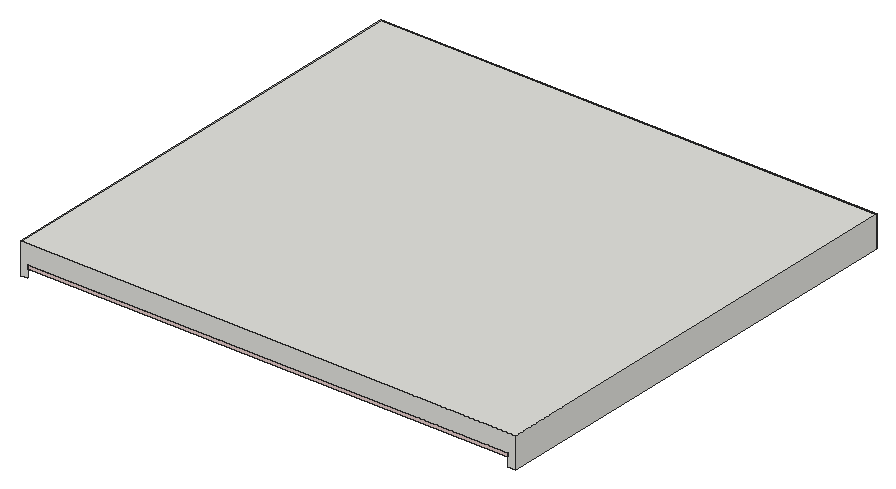
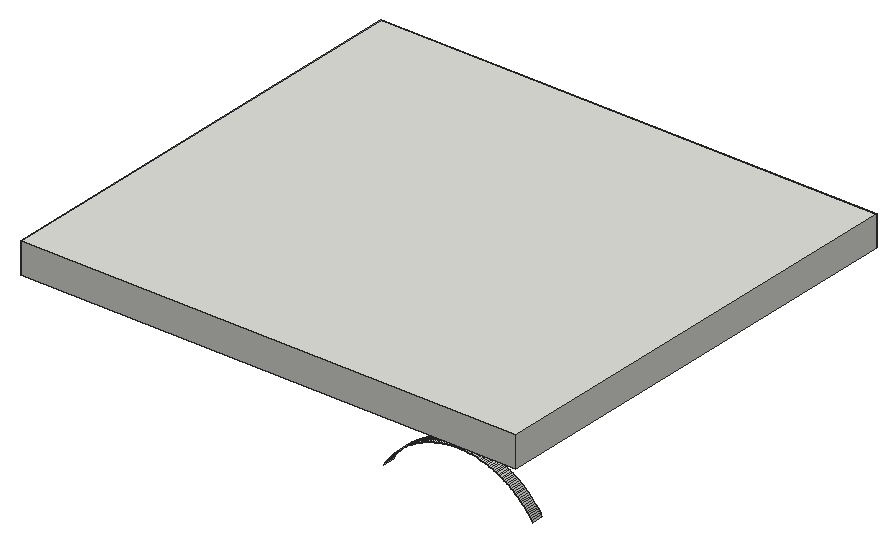
# SketchUp Ruby script. Lengths in inches.
U = 1.inch
M = Sketchup.active_model
def pt(a) = Geom::Point3d.new(a.map { |v| v * U })
def face(e, loops, mat)
  f = e.add_face(loops[0].map { |a| pt(a) })
  loops[1..].each { |l| e.add_face(l.map { |a| pt(a) }).erase! }
  f.material = f.back_material = mat if mat
  f
end
# faces: each face lists its corners as indices into pts; further lists are holes
def faces(e, pts, list, mat = nil) = list.each { |f| face(e, (f[0].is_a?(Array) ? f : [f]).map { |l| l.map { |i| pts[i] } }, mat) }
# xy, xz, yz: faces in a plane at the given z, y or x. An outline is a flat list of corners, or four numbers for a rectangle; further outlines are holes
def ring(l) = l.size == 4 ? [[l[0], l[1]], [l[2], l[1]], [l[2], l[3]], [l[0], l[3]]] : l.each_slice(2).to_a
def flat(e, list, mat, &to3) = list.each { |f| face(e, (f[0].is_a?(Array) ? f : [f]).map { |l| ring(l).map { |u, v| to3.(u, v) } }, mat) }
def xy(e, z, list, mat = nil) = flat(e, list, mat) { |x, y| [x, y, z] }
def xz(e, y, list, mat = nil) = flat(e, list, mat) { |x, z| [x, y, z] }
def yz(e, x, list, mat = nil) = flat(e, list, mat) { |y, z| [x, y, z] }
def lines(e, pts, list) = list.each { |a, b| e.add_line(pt(pts[a]), pt(pts[b])) }
# prism: a flat outline (further loops are holes) pulled along v
def prism(e, loops, v, mat = nil)
  f = face(e, loops, mat); d = Geom::Vector3d.new(v.map { |x| x * U })
  f.pushpull(f.normal.samedirection?(d) ? d.length : -d.length)
end
def box(e, o, s, mat = nil) = prism(e, [[o, [o[0] + s[0], o[1], o[2]], [o[0] + s[0], o[1] + s[1], o[2]], [o[0], o[1] + s[1], o[2]]]], [0, 0, s[2]], mat)
def at(x, y, z, deg = 0) = Geom::Transformation.translation(pt([x, y, z])) * Geom::Transformation.rotation(ORIGIN, Z_AXIS, deg.degrees)
def axes(o, x, y, z) = Geom::Transformation.new([*x, 0, *y, 0, *z, 0, *pt(o).to_a, 1])
def part(name) = M.definitions.add(name)
# library, detail: a bought-in or finely detailed component or shape, given as its bounding box
def library(name, o, s) = part(name).tap { |d| box(d.entities, o, s) }
def detail(e, o, s) = box(e.add_group.entities, o, s)
def put(e, d, t, mat = nil) = e.add_instance(d, t).tap { |i| i.material = mat if mat }
def group(e, t, mat = nil) = e.add_group.tap { |g| g.transformation = t; g.material = mat if mat }.entities
root = M.entities
M.materials.add("[0007_MistyRose]").color = [232, 207, 204]
M.materials.add("[0134_DimGray]").color = [105, 105, 105]
xy(root,122.125,[[77.27,180.253,114.094,204.253],[114.394,180.253,114.394,180.378,114.094,180.378,114.094,204.253,150.918,204.253,150.918,180.253],[150.918,180.253,150.918,204.253,187.741,204.253,187.741,183.815,169.329,183.815,169.329,180.253],[169.329,180.253,187.741,183.815],[188.041,180.253,208.642,180.378],
  [208.642,180.253,224.565,180.378],[187.741,180.378,224.565,204.253],[3.622,184.565,40.446,189.878],[40.446,184.565,77.27,204.253],[3.622,189.878,40.446,204.253]])
xy(root,127.75,[[3.435,0,3.435,93.375,3.622,204.253,3.622,189.878,40.446,189.878,40.446,184.565,77.27,184.565,77.27,180.253,114.094,180.253,114.094,180.378,114.394,180.378,114.394,180.253,169.329,180.253,169.329,183.815,187.741,183.815,187.741,180.378,224.565,180.378,224.565,0]])
xy(root,136.1875,[[0,0,228,207.6875]])
xz(root,0,[[0,122.125,3.435,122.125,3.435,127.75,224.565,127.75,224.565,122.125,228,122.125,228,136.1875,0,136.1875]])
xz(root,180.253,[[77.27,122.125,95.682,127.75],[95.682,122.125,114.094,127.75],[114.394,122.125,133.557,127.75],[133.557,122.125,150.918,127.75],[150.918,122.125,151.218,127.75],
  [151.218,122.125,169.329,127.75]])
xz(root,180.378,[[114.094,122.125,114.394,127.75],[187.741,122.125,188.041,127.75]])
xz(root,180.378,[[188.041,122.125,224.565,127.75]],"[0134_DimGray]")
xz(root,183.815,[[169.329,122.125,187.741,127.75]],"[0134_DimGray]")
xz(root,184.565,[[40.446,122.125,77.27,127.75]],"[0134_DimGray]")
xz(root,189.878,[[3.622,122.125,40.446,127.75]],"[0134_DimGray]")
xz(root,207.6875,[[0,122.125,228,136.1875]])
yz(root,0,[[0,122.125,207.6875,136.1875]])
yz(root,3.622,[[189.878,122.125,204.253,127.75]])
yz(root,40.446,[[184.565,122.125,189.878,127.75]])
yz(root,77.27,[[180.253,122.125,184.565,127.75]])
yz(root,114.094,[[180.253,122.125,180.378,127.75]])
yz(root,114.394,[[180.253,122.125,180.378,127.75]])
yz(root,169.329,[[180.253,122.125,183.815,127.75]])
yz(root,187.741,[[180.378,122.125,183.815,127.75]])
yz(root,228,[[0,122.125,207.6875,136.1875]])
p = [[6.197,184.565,90.119],[6.197,190.128,90.119],[6.615,190.128,90.765],[6.615,184.565,90.765],[74.277,184.565,90.765],[74.277,190.128,90.765],
  [74.695,190.128,90.119],[74.695,184.565,90.119],[7.046,190.128,91.403],[7.046,184.565,91.403],[73.847,184.565,91.403],[73.847,190.128,91.403],
  [7.488,190.128,92.033],[7.488,184.565,92.033],[73.404,184.565,92.033],[73.404,190.128,92.033],[7.942,190.128,92.654],[7.942,184.565,92.654],
  [72.95,184.565,92.654],[72.95,190.128,92.654],[8.408,190.128,93.266],[8.408,184.565,93.266],[72.484,184.565,93.266],[72.484,190.128,93.266],
  [8.886,190.128,93.869],[8.886,184.565,93.869],[72.006,184.565,93.869],[72.006,190.128,93.869],[9.375,190.128,94.464],[9.375,184.565,94.464],
  [71.517,184.565,94.464],[71.517,190.128,94.464],[9.875,190.128,95.048],[9.875,184.565,95.048],[71.017,184.565,95.048],[71.017,190.128,95.048],
  [10.386,190.128,95.624],[10.386,184.565,95.624],[70.506,184.565,95.624],[70.506,190.128,95.624],[10.908,190.128,96.189],[10.908,184.565,96.189],
  [69.984,184.565,96.189],[69.984,190.128,96.189],[11.441,190.128,96.744],[11.441,184.565,96.744],[69.452,184.565,96.744],[69.452,190.128,96.744],
  [11.984,190.128,97.29],[11.984,184.565,97.29],[68.909,184.565,97.29],[68.909,190.128,97.29],[12.537,190.128,97.824],[12.537,184.565,97.824],
  [68.355,184.565,97.824],[68.355,190.128,97.824],[13.1,190.128,98.349],[13.1,184.565,98.349],[67.792,184.565,98.349],[67.792,190.128,98.349],
  [13.673,190.128,98.862],[13.673,184.565,98.862],[67.219,184.565,98.862],[67.219,190.128,98.862],[14.256,190.128,99.365],[14.256,184.565,99.365],
  [66.636,184.565,99.365],[66.636,190.128,99.365],[14.848,190.128,99.856],[14.848,184.565,99.856],[66.044,184.565,99.856],[66.044,190.128,99.856],
  [15.45,190.128,100.336],[15.45,184.565,100.336],[65.442,184.565,100.336],[65.442,190.128,100.336],[16.06,190.128,100.804],[16.06,184.565,100.804],
  [64.832,184.565,100.804],[64.832,190.128,100.804],[16.679,190.128,101.261],[16.679,184.565,101.261],[64.213,184.565,101.261],[64.213,190.128,101.261],
  [17.307,190.128,101.706],[17.307,184.565,101.706],[63.585,184.565,101.706],[63.585,190.128,101.706],[17.943,190.128,102.139],[17.943,184.565,102.139],
  [62.949,184.565,102.139],[62.949,190.128,102.139],[18.588,190.128,102.56],[18.588,184.565,102.56],[62.305,184.565,102.56],[62.305,190.128,102.56],
  [19.24,190.128,102.969],[19.24,184.565,102.969],[61.653,184.565,102.969],[61.653,190.128,102.969],[19.899,190.128,103.365],[19.899,184.565,103.365],
  [60.993,184.565,103.365],[60.993,190.128,103.365],[20.566,190.128,103.748],[20.566,184.565,103.748],[60.326,184.565,103.748],[60.326,190.128,103.748],
  [21.241,190.128,104.119],[21.241,184.565,104.119],[59.652,184.565,104.119],[59.652,190.128,104.119],[21.922,190.128,104.477],[21.922,184.565,104.477],
  [58.97,184.565,104.477],[58.97,190.128,104.477],[22.61,190.128,104.822],[22.61,184.565,104.822],[58.283,184.565,104.822],[58.283,190.128,104.822],
  [23.304,190.128,105.154],[23.304,184.565,105.154],[57.588,184.565,105.154],[57.588,190.128,105.154],[24.004,190.128,105.473],[24.004,184.565,105.473],
  [56.888,184.565,105.473],[56.888,190.128,105.473],[24.711,190.128,105.778],[24.711,184.565,105.778],[56.181,184.565,105.778],[56.181,190.128,105.778],
  [25.423,190.128,106.07],[25.423,184.565,106.07],[55.469,184.565,106.07],[55.469,190.128,106.07],[26.14,190.128,106.348],[26.14,184.565,106.348],
  [54.752,184.565,106.348],[54.752,190.128,106.348],[26.863,190.128,106.612],[26.863,184.565,106.612],[54.029,184.565,106.612],[54.029,190.128,106.612],
  [27.59,190.128,106.863],[27.59,184.565,106.863],[53.302,184.565,106.863],[53.302,190.128,106.863],[28.322,190.128,107.1],[28.322,184.565,107.1],
  [52.57,184.565,107.1],[52.57,190.128,107.1],[29.059,190.128,107.323],[29.059,184.565,107.323],[51.833,184.565,107.323],[51.833,190.128,107.323],
  [29.799,190.128,107.532],[29.799,184.565,107.532],[51.093,184.565,107.532],[51.093,190.128,107.532],[30.544,190.128,107.727],[30.544,184.565,107.727],
  [50.349,184.565,107.727],[50.349,190.128,107.727],[31.292,190.128,107.908],[31.292,184.565,107.908],[49.601,184.565,107.908],[49.601,190.128,107.908],
  [32.043,190.128,108.075],[32.043,184.565,108.075],[48.849,184.565,108.075],[48.849,190.128,108.075],[32.797,190.128,108.227],[32.797,184.565,108.227],
  [48.095,184.565,108.227],[48.095,190.128,108.227],[33.554,190.128,108.365],[33.554,184.565,108.365],[47.338,184.565,108.365],[47.338,190.128,108.365],
  [34.314,190.128,108.489],[34.314,184.565,108.489],[46.579,184.565,108.489],[46.579,190.128,108.489],[35.075,190.128,108.598],[35.075,184.565,108.598],
  [45.817,184.565,108.598],[45.817,190.128,108.598],[35.839,190.128,108.692],[35.839,184.565,108.692],[45.053,184.565,108.692],[45.053,190.128,108.692],
  [36.604,190.128,108.773],[36.604,184.565,108.773],[44.288,184.565,108.773],[44.288,190.128,108.773],[37.371,190.128,108.838],[37.371,184.565,108.838],
  [38.139,190.128,108.889],[38.139,184.565,108.889],[42.753,184.565,108.889],[42.753,190.128,108.889],[43.521,190.128,108.838],[43.521,184.565,108.838],
  [38.907,190.128,108.926],[38.907,184.565,108.926],[39.677,190.128,108.948],[39.677,184.565,108.948],[40.446,190.128,108.955],[40.446,184.565,108.955],
  [40.746,190.128,108.952],[41.216,190.128,108.948],[41.216,184.565,108.948],[41.985,190.128,108.926],[41.985,184.565,108.926],[40.746,190.128,108.955]]
faces(root,p,[[0,1,2,3],[4,5,6,7],[3,2,8,9],[10,11,5,4],[9,8,12,13],[14,15,11,10],[13,12,16,17],[18,19,15,14],
  [17,16,20,21],[22,23,19,18],[21,20,24,25],[26,27,23,22],[25,24,28,29],[30,31,27,26],[29,28,32,33],[34,35,31,30],
  [33,32,36,37],[38,39,35,34],[37,36,40,41],[42,43,39,38],[41,40,44,45],[46,47,43,42],[45,44,48,49],[50,51,47,46],
  [49,48,52,53],[54,55,51,50],[53,52,56,57],[58,59,55,54],[57,56,60,61],[62,63,59,58],[61,60,64,65],[66,67,63,62],
  [65,64,68,69],[70,71,67,66],[69,68,72,73],[74,75,71,70],[73,72,76,77],[78,79,75,74],[77,76,80,81],[82,83,79,78],
  [81,80,84,85],[86,87,83,82],[85,84,88,89],[90,91,87,86],[89,88,92,93],[94,95,91,90],[93,92,96,97],[98,99,95,94],
  [97,96,100,101],[102,103,99,98],[101,100,104,105],[106,107,103,102],[105,104,108,109],[110,111,107,106],[109,108,112,113],[114,115,111,110],
  [113,112,116,117],[118,119,115,114],[117,116,120,121],[122,123,119,118],[121,120,124,125],[126,127,123,122],[125,124,128,129],[130,131,127,126],
  [129,128,132,133],[134,135,131,130],[133,132,136,137],[138,139,135,134],[137,136,140,141],[142,143,139,138],[141,140,144,145],[146,147,143,142],
  [145,144,148,149],[150,151,147,146],[149,148,152,153],[154,155,151,150],[153,152,156,157],[158,159,155,154],[157,156,160,161],[162,163,159,158],
  [161,160,164,165],[166,167,163,162],[165,164,168,169],[170,171,167,166],[169,168,172,173],[174,175,171,170],[173,172,176,177],[178,179,175,174],
  [177,176,180,181],[182,183,179,178],[181,180,184,185],[186,187,183,182],[185,184,188,189],[190,191,187,186],[189,188,192,193],[194,195,191,190],
  [193,192,196,197],[197,196,198,199],[200,201,202,203],[203,202,195,194],[199,198,204,205],[205,204,206,207],[207,206,208,209],[209,208,210,211,212],
  [212,211,213,214],[214,213,201,200]])
lines(root,p,[[210,215]])
g1 = group(root,at(3.43,0,122.3125),"[0007_MistyRose]")
xy(g1,0,[[[107.92,50.6,101.84,51.04,95.82,51.92,89.875,53.26,84.05,55.04,78.37,57.24,72.87,59.87,67.59,62.9,62.54,66.32,57.77,70.11,53.3,74.24,49.14,78.69,45.33,83.45,41.89,88.48,38.84,93.75,36.18,99.23,33.95,104.9,32.14,110.72,30.78,116.65,29.87,122.68,29.4,128.75,29.4,134.84,29.85,140.92,30.75,146.94,32.11,152.88,33.9,158.7,36.125,164.375,38.77,169.86,41.8125,175.14,45.24,180.17,49.47,184.57,73.84,184.57,73.84,180.25,110.66,180.25,110.66,180.38,110.96,180.38,110.96,180.25,175.15,180.25,179.18,175.66,182.26,170.41,184.95,164.9375,187.21,159.28,189.05,153.48,190.45,147.55,191.4,141.53,191.89,135.46,191.93,129.37,191.52,123.29,190.65,117.26,189.33,111.3125,187.57,105.48,185.38,99.79,182.77,94.29,179.75,89,176.35,83.95,172.58,79.16,168.46,74.67,164.01,70.51,159.27,66.6875,154.25,63.23,148.99,60.16,143.51,57.49,137.85,55.24,132.04,53.42,126.11,52.04,120.09,51.11,114.01,50.625],[110.64,167.88,111.11,167.94,111.55,168.125,111.92,168.41,112.21,168.79,112.39,169.22,112.45,169.69,112.39,170.16,112.21,170.6,111.92,170.98,111.55,171.26,111.11,171.45,110.64,171.51,110.17,171.45,109.73,171.26,109.36,170.98,109.07,170.6,108.89,170.16,108.83,169.69,108.89,169.22,109.07,168.79,109.36,168.41,109.73,168.125,110.17,167.94],[107.125,168.01,107.5625,168.0625,107.97,168.23,108.32,168.5,108.59,168.85,108.75,169.26,108.8125,169.69,108.75,170.13,108.59,170.54,108.32,170.89,107.97,171.16,107.5625,171.32,107.125,171.38,106.6875,171.32,106.28,171.16,105.93,170.89,105.66,170.54,105.49,170.13,105.4375,169.69,105.49,169.26,105.66,168.85,105.93,168.5,106.28,168.23,106.6875,168.0625]],[110.64,167.88,110.17,167.94,109.73,168.125,109.36,168.41,109.07,168.79,108.89,169.22,108.83,169.69,108.89,170.16,109.07,170.6,109.36,170.98,109.73,171.26,110.17,171.45,110.64,171.51,111.11,171.45,111.55,171.26,111.92,170.98,112.21,170.6,112.39,170.16,112.45,169.69,112.39,169.22,112.21,168.79,111.92,168.41,111.55,168.125,111.11,167.94],[107.125,168.01,106.6875,168.0625,106.28,168.23,105.93,168.5,105.66,168.85,105.49,169.26,105.4375,169.69,105.49,170.13,105.66,170.54,105.93,170.89,106.28,171.16,106.6875,171.32,107.125,171.38,107.5625,171.32,107.97,171.16,108.32,170.89,108.59,170.54,108.75,170.13,108.8125,169.69,108.75,169.26,108.59,168.85,108.32,168.5,107.97,168.23,107.5625,168.0625]])
xy(g1,2.6875,[[10.36,78.8,9.68,78.89,9.05,79.15,8.51,79.57,8.09,80.11,7.83,80.75,7.74,81.43,7.83,82.11,8.09,82.74,8.51,83.28,9.05,83.7,9.68,83.96,10.36,84.05,11.04,83.96,11.68,83.7,12.22,83.28,12.64,82.74,12.9,82.11,12.99,81.43,12.9,80.75,12.64,80.11,12.22,79.57,11.68,79.15,11.04,78.89],[211.55,78.8,210.87,78.89,210.24,79.15,209.7,79.57,209.28,80.11,209.02,80.75,208.93,81.43,209.02,82.11,209.28,82.74,209.7,83.28,210.24,83.7,210.87,83.96,211.55,84.05,212.23,83.96,212.86,83.7,213.41,83.28,213.83,82.74,214.09,82.11,214.18,81.43,214.09,80.75,213.83,80.11,213.41,79.57,212.86,79.15,212.23,78.89]])
xy(g1,3.75,[[[0,0,0,93.375,0.1875,204.25,0.1875,184.57,49.47,184.57,45.24,180.17,41.8125,175.14,38.77,169.86,36.125,164.375,33.9,158.7,32.11,152.88,30.75,146.94,29.85,140.92,29.4,134.84,29.4,128.75,29.87,122.68,30.78,116.65,32.14,110.72,33.95,104.9,36.18,99.23,38.84,93.75,41.89,88.48,45.33,83.45,49.14,78.69,53.3,74.24,57.77,70.11,62.54,66.32,67.59,62.9,72.87,59.87,78.37,57.24,84.05,55.04,89.875,53.26,95.82,51.92,101.84,51.04,107.92,50.6,114.01,50.625,120.09,51.11,126.11,52.04,132.04,53.42,137.85,55.24,143.51,57.49,148.99,60.16,154.25,63.23,159.27,66.6875,164.01,70.51,168.46,74.67,172.58,79.16,176.35,83.95,179.75,89,182.77,94.29,185.38,99.79,187.57,105.48,189.33,111.3125,190.65,117.26,191.52,123.29,191.93,129.37,191.89,135.46,191.4,141.53,190.45,147.55,189.05,153.48,187.21,159.28,184.95,164.9375,182.26,170.41,179.18,175.66,175.15,180.25,184.31,180.25,184.31,180.38,184.61,180.38,184.61,180.25,221.13,180.25,221.13,0],[211.55,78.8,212.23,78.89,212.86,79.15,213.41,79.57,213.83,80.11,214.09,80.75,214.18,81.43,214.09,82.11,213.83,82.74,213.41,83.28,212.86,83.7,212.23,83.96,211.55,84.05,210.87,83.96,210.24,83.7,209.7,83.28,209.28,82.74,209.02,82.11,208.93,81.43,209.02,80.75,209.28,80.11,209.7,79.57,210.24,79.15,210.87,78.89],[10.36,78.8,11.04,78.89,11.68,79.15,12.22,79.57,12.64,80.11,12.9,80.75,12.99,81.43,12.9,82.11,12.64,82.74,12.22,83.28,11.68,83.7,11.04,83.96,10.36,84.05,9.68,83.96,9.05,83.7,8.51,83.28,8.09,82.74,7.83,82.11,7.74,81.43,7.83,80.75,8.09,80.11,8.51,79.57,9.05,79.15,9.68,78.89]]])
xz(g1,0,[[0,3.75,221.13,5.4375]])
xz(g1,180.25,[[73.84,0,92.25,5.4375],[92.25,0,110.66,5.4375],[110.96,0,130.12,5.4375],[130.12,0,147.48,5.4375],[147.48,0,147.78,5.4375],
  [147.78,0,165.89,5.4375],[165.89,0,175.15,5.4375],[175.15,3.75,184.31,5.4375],[184.61,3.75,205.21,5.4375],[205.21,3.75,221.13,5.4375]])
xz(g1,180.38,[[110.66,0,110.96,5.4375],[184.31,3.75,184.61,5.4375]])
xz(g1,184.57,[[49.47,0,73.84,5.4375],[0.1875,3.75,37.01,5.4375],[37.01,3.75,49.47,5.4375]])
yz(g1,0,[[0,3.75,93.375,5.4375]])
yz(g1,0.1875,[[184.57,3.75,204.25,5.4375]])
yz(g1,29.4,[[128.75,0,134.84,3.75]])
yz(g1,73.84,[[180.25,0,184.57,5.4375]])
yz(g1,110.66,[[180.25,0,180.38,5.4375]])
yz(g1,110.96,[[180.25,0,180.38,5.4375]])
yz(g1,184.31,[[180.25,3.75,180.38,5.4375]])
yz(g1,184.61,[[180.25,3.75,180.38,5.4375]])
yz(g1,221.13,[[0,3.75,180.25,5.4375]])
p = [[107.92,50.6,0],[107.92,50.6,3.75],[101.84,51.04,3.75],[101.84,51.04,0],[114.01,50.625,0],[114.01,50.625,3.75],
  [120.09,51.11,0],[120.09,51.11,3.75],[95.82,51.92,3.75],[95.82,51.92,0],[126.11,52.04,0],[126.11,52.04,3.75],
  [89.875,53.26,3.75],[89.875,53.26,0],[132.04,53.42,0],[132.04,53.42,3.75],[84.05,55.04,3.75],[84.05,55.04,0],
  [137.85,55.24,0],[137.85,55.24,3.75],[78.37,57.24,3.75],[78.37,57.24,0],[143.51,57.49,0],[143.51,57.49,3.75],
  [72.87,59.87,3.75],[72.87,59.87,0],[148.99,60.16,0],[148.99,60.16,3.75],[67.59,62.9,3.75],[67.59,62.9,0],
  [154.25,63.23,0],[154.25,63.23,3.75],[62.54,66.32,3.75],[62.54,66.32,0],[159.27,66.6875,0],[159.27,66.6875,3.75],
  [57.77,70.11,3.75],[57.77,70.11,0],[164.01,70.51,0],[164.01,70.51,3.75],[53.3,74.24,3.75],[53.3,74.24,0],
  [168.46,74.67,0],[168.46,74.67,3.75],[49.14,78.69,3.75],[49.14,78.69,0],[172.58,79.16,0],[172.58,79.16,3.75],
  [45.33,83.45,3.75],[45.33,83.45,0],[176.35,83.95,0],[176.35,83.95,3.75],[41.89,88.48,3.75],[41.89,88.48,0],
  [179.75,89,0],[179.75,89,3.75],[38.84,93.75,3.75],[38.84,93.75,0],[182.77,94.29,0],[182.77,94.29,3.75],
  [36.18,99.23,3.75],[36.18,99.23,0],[185.38,99.79,0],[185.38,99.79,3.75],[33.95,104.9,3.75],[33.95,104.9,0],
  [187.57,105.48,0],[187.57,105.48,3.75],[32.14,110.72,3.75],[32.14,110.72,0],[189.33,111.3125,0],[189.33,111.3125,3.75],
  [30.78,116.65,3.75],[30.78,116.65,0],[190.65,117.26,0],[190.65,117.26,3.75],[29.87,122.68,3.75],[29.87,122.68,0],
  [191.52,123.29,0],[191.52,123.29,3.75],[29.4,128.75,3.75],[29.4,128.75,0],[191.93,129.37,0],[191.93,129.37,3.75],
  [191.89,135.46,0],[191.89,135.46,3.75],[29.4,134.84,0],[29.4,134.84,3.75],[29.85,140.92,3.75],[29.85,140.92,0],
  [191.4,141.53,0],[191.4,141.53,3.75],[30.75,146.94,3.75],[30.75,146.94,0],[190.45,147.55,0],[190.45,147.55,3.75],
  [32.11,152.88,3.75],[32.11,152.88,0],[189.05,153.48,0],[189.05,153.48,3.75],[33.9,158.7,3.75],[33.9,158.7,0],
  [187.21,159.28,0],[187.21,159.28,3.75],[36.125,164.375,3.75],[36.125,164.375,0],[184.95,164.9375,0],[184.95,164.9375,3.75],
  [38.77,169.86,3.75],[38.77,169.86,0],[182.26,170.41,0],[182.26,170.41,3.75],[41.8125,175.14,3.75],[41.8125,175.14,0],
  [179.18,175.66,0],[179.18,175.66,3.75],[45.24,180.17,3.75],[45.24,180.17,0],[175.15,180.25,0],[175.15,180.25,3.75],
  [49.47,184.57,3.75],[49.47,184.57,0],[10.36,78.8,3.75],[9.68,78.89,3.75],[9.68,78.89,2.6875],[10.36,78.8,2.6875],
  [11.04,78.89,3.75],[11.04,78.89,2.6875],[211.55,78.8,3.75],[210.87,78.89,3.75],[210.87,78.89,2.6875],[211.55,78.8,2.6875],
  [212.23,78.89,3.75],[212.23,78.89,2.6875],[9.05,79.15,3.75],[9.05,79.15,2.6875],[11.68,79.15,3.75],[11.68,79.15,2.6875],
  [210.24,79.15,3.75],[210.24,79.15,2.6875],[212.86,79.15,3.75],[212.86,79.15,2.6875],[8.51,79.57,3.75],[8.51,79.57,2.6875],
  [12.22,79.57,3.75],[12.22,79.57,2.6875],[209.7,79.57,3.75],[209.7,79.57,2.6875],[213.41,79.57,3.75],[213.41,79.57,2.6875],
  [8.09,80.11,3.75],[8.09,80.11,2.6875],[12.64,80.11,3.75],[12.64,80.11,2.6875],[209.28,80.11,3.75],[209.28,80.11,2.6875],
  [213.83,80.11,3.75],[213.83,80.11,2.6875],[7.83,80.75,3.75],[7.83,80.75,2.6875],[12.9,80.75,3.75],[12.9,80.75,2.6875],
  [209.02,80.75,3.75],[209.02,80.75,2.6875],[214.09,80.75,3.75],[214.09,80.75,2.6875],[7.74,81.43,3.75],[7.74,81.43,2.6875],
  [12.99,81.43,3.75],[12.99,81.43,2.6875],[208.93,81.43,3.75],[208.93,81.43,2.6875],[214.18,81.43,3.75],[214.18,81.43,2.6875],
  [7.83,82.11,3.75],[7.83,82.11,2.6875],[12.9,82.11,3.75],[12.9,82.11,2.6875],[209.02,82.11,3.75],[209.02,82.11,2.6875],
  [214.09,82.11,3.75],[214.09,82.11,2.6875],[8.09,82.74,3.75],[8.09,82.74,2.6875],[12.64,82.74,3.75],[12.64,82.74,2.6875],
  [209.28,82.74,3.75],[209.28,82.74,2.6875],[213.83,82.74,3.75],[213.83,82.74,2.6875],[8.51,83.28,3.75],[8.51,83.28,2.6875],
  [12.22,83.28,3.75],[12.22,83.28,2.6875],[209.7,83.28,3.75],[209.7,83.28,2.6875],[213.41,83.28,3.75],[213.41,83.28,2.6875],
  [9.05,83.7,3.75],[9.05,83.7,2.6875],[11.68,83.7,3.75],[11.68,83.7,2.6875],[210.24,83.7,3.75],[210.24,83.7,2.6875],
  [212.86,83.7,3.75],[212.86,83.7,2.6875],[9.68,83.96,3.75],[9.68,83.96,2.6875],[11.04,83.96,3.75],[11.04,83.96,2.6875],
  [210.87,83.96,3.75],[210.87,83.96,2.6875],[212.23,83.96,3.75],[212.23,83.96,2.6875],[10.36,84.05,3.75],[10.36,84.05,2.6875],
  [211.55,84.05,3.75],[211.55,84.05,2.6875],[0,93.375,5.4375],[0.1875,204.25,5.4375],[0.1875,204.25,3.75],[0,93.375,3.75]]
faces(g1,p,[[0,1,2,3],[4,5,1,0],[6,7,5,4],[3,2,8,9],[10,11,7,6],[9,8,12,13],[14,15,11,10],[13,12,16,17],
  [18,19,15,14],[17,16,20,21],[22,23,19,18],[21,20,24,25],[26,27,23,22],[25,24,28,29],[30,31,27,26],[29,28,32,33],
  [34,35,31,30],[33,32,36,37],[38,39,35,34],[37,36,40,41],[42,43,39,38],[41,40,44,45],[46,47,43,42],[45,44,48,49],
  [50,51,47,46],[49,48,52,53],[54,55,51,50],[53,52,56,57],[58,59,55,54],[57,56,60,61],[62,63,59,58],[61,60,64,65],
  [66,67,63,62],[65,64,68,69],[70,71,67,66],[69,68,72,73],[74,75,71,70],[73,72,76,77],[78,79,75,74],[77,76,80,81],
  [82,83,79,78],[84,85,83,82],[86,87,88,89],[90,91,85,84],[89,88,92,93],[94,95,91,90],[93,92,96,97],[98,99,95,94],
  [97,96,100,101],[102,103,99,98],[101,100,104,105],[106,107,103,102],[105,104,108,109],[110,111,107,106],[109,108,112,113],[114,115,111,110],
  [113,112,116,117],[118,119,115,114],[117,116,120,121],[122,123,124,125],[126,122,125,127],[128,129,130,131],[132,128,131,133],[123,134,135,124],
  [136,126,127,137],[129,138,139,130],[140,132,133,141],[134,142,143,135],[144,136,137,145],[138,146,147,139],[148,140,141,149],[142,150,151,143],
  [152,144,145,153],[146,154,155,147],[156,148,149,157],[150,158,159,151],[160,152,153,161],[154,162,163,155],[164,156,157,165],[158,166,167,159],
  [168,160,161,169],[162,170,171,163],[172,164,165,173],[166,174,175,167],[176,168,169,177],[170,178,179,171],[180,172,173,181],[174,182,183,175],
  [184,176,177,185],[178,186,187,179],[188,180,181,189],[182,190,191,183],[192,184,185,193],[186,194,195,187],[196,188,189,197],[190,198,199,191],
  [200,192,193,201],[194,202,203,195],[204,196,197,205],[198,206,207,199],[208,200,201,209],[202,210,211,203],[212,204,205,213],[206,214,215,207],
  [214,208,209,215],[210,216,217,211],[216,212,213,217],[218,219,220,221]])
